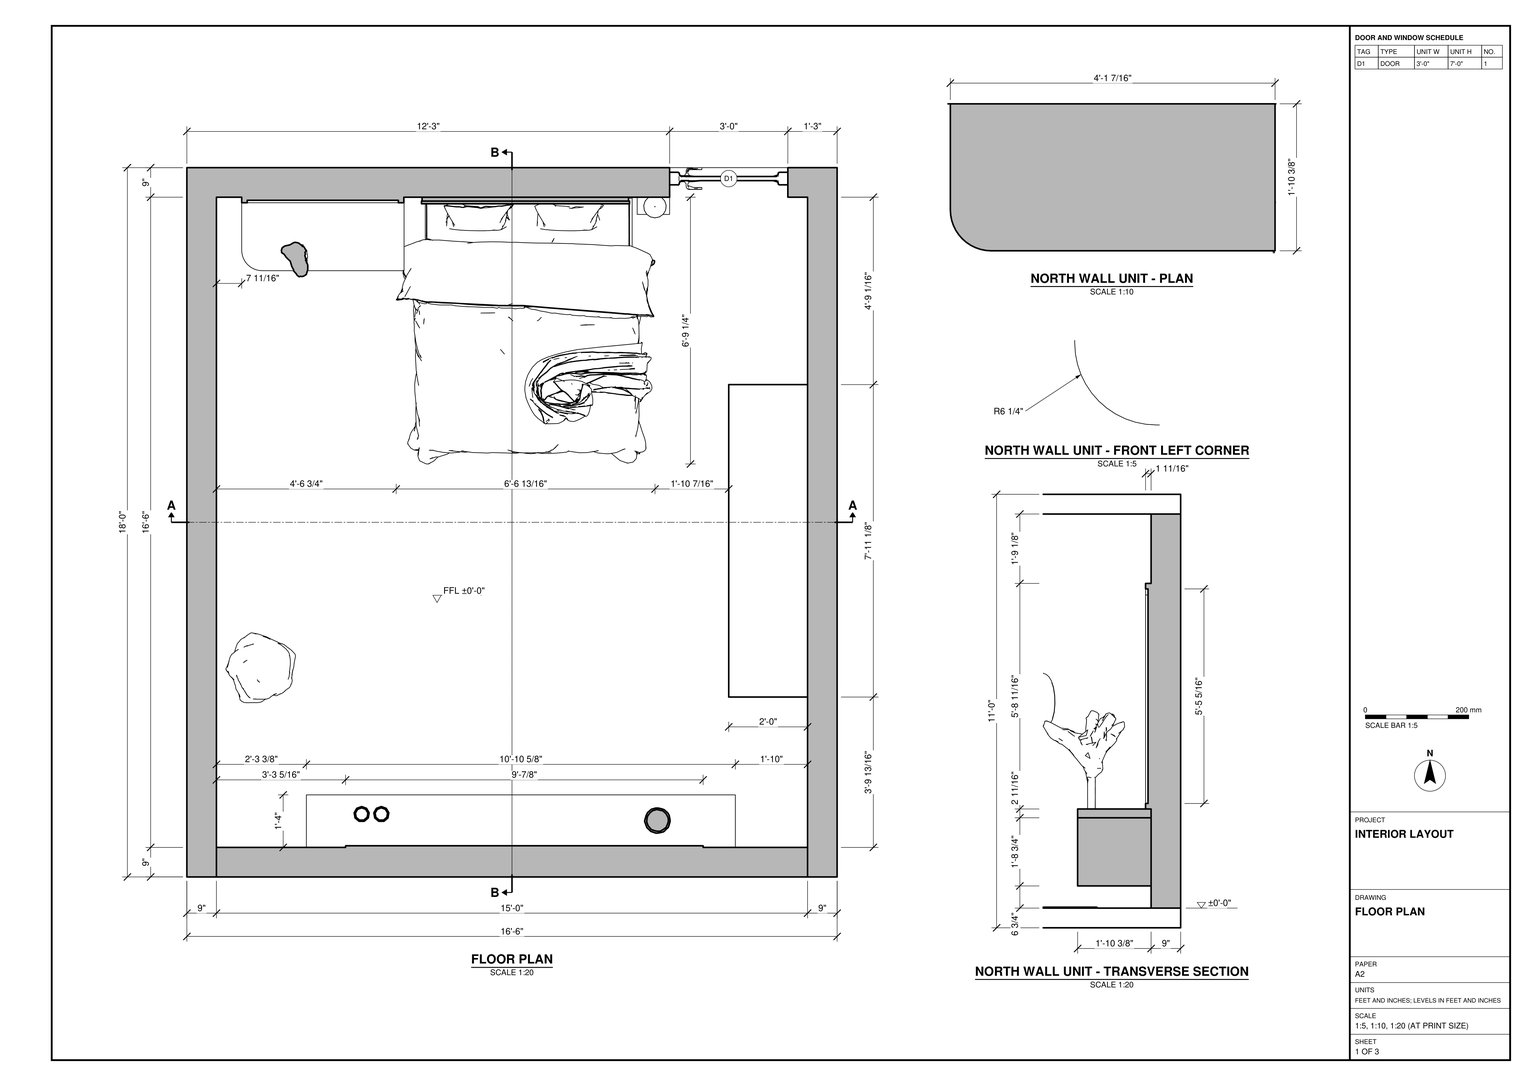
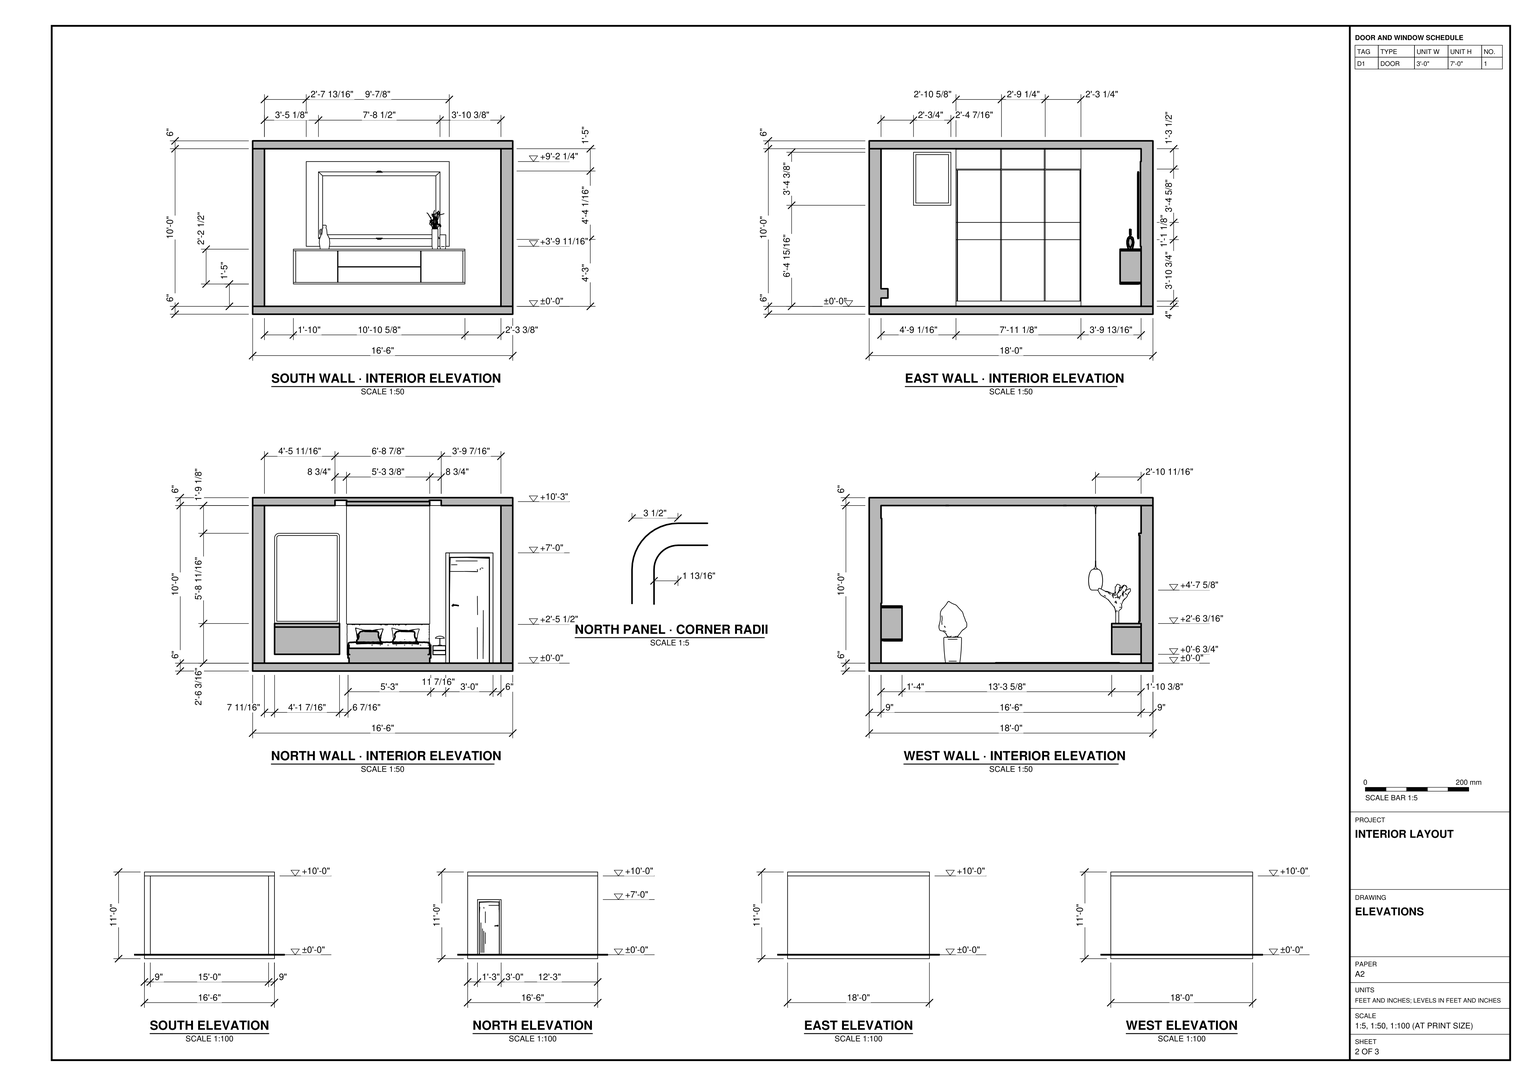
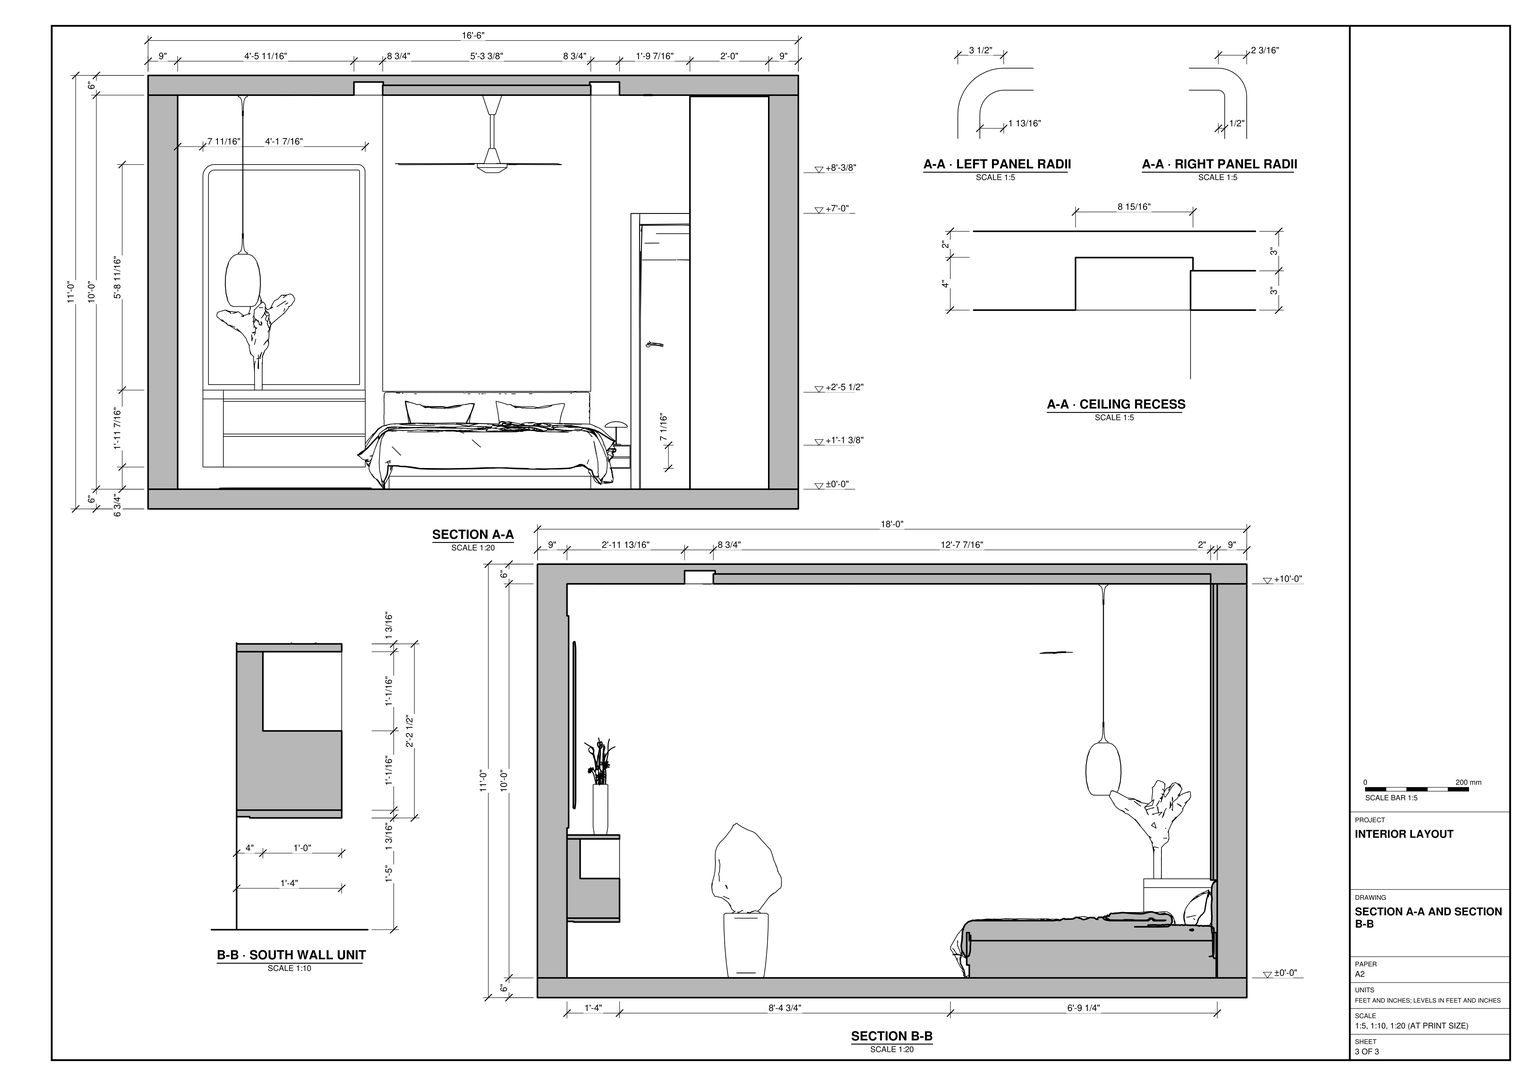
Build the bedroom in SketchUp from task_files/diagram_01.pdf. Work in feet and inches. The room shell measures 16'-6" east to west by 18'-0" north to south, with an overall height of 11'-0". Use the finished floor at ±0'-0" as the single storey level. Model the 9" perimeter walls, the 6" floor and roof slabs, and the stepped recess in the ceiling shown in sections A-A and B-B. Place the 3'-0" by 7'-0" entrance door near the east end of the north wall.

Set the platform bed with its head against the north wall. Align the tall panel behind the headboard with the ceiling detail. To the left of the bed, model the suspended cabinet with its rounded front-left corner and the framed panel above it. Include the small bedside unit on the door side. Use the east elevation to lay out the divisions on the full-height storage unit. Opposite the bed, model the floating south wall cabinet with its shelving and the framed rectangular panel above it. Place the ceiling fan, pendant, floor plant and tabletop objects where shown. Decor and loose items may be any suitable library components.

Keep the walls, floor slab and roof separate, and make each furniture or joinery piece a separate group or component. Use components for repeated parts. Save one SketchUp model as output_files/bedroom_with_fitted_wall_units_and_a_recessed_ceiling.skp.

# SketchUp Ruby script. Lengths in inches.
U = 1.inch
M = Sketchup.active_model
def pt(a) = Geom::Point3d.new(a.map { |v| v * U })
def face(e, loops, mat)
  f = e.add_face(loops[0].map { |a| pt(a) })
  loops[1..].each { |l| e.add_face(l.map { |a| pt(a) }).erase! }
  f.material = f.back_material = mat if mat
  f
end
# faces: each face lists its corners as indices into pts; further lists are holes
def faces(e, pts, list, mat = nil) = list.each { |f| face(e, (f[0].is_a?(Array) ? f : [f]).map { |l| l.map { |i| pts[i] } }, mat) }
# xy, xz, yz: faces in a plane at the given z, y or x. An outline is a flat list of corners, or four numbers for a rectangle; further outlines are holes
def ring(l) = l.size == 4 ? [[l[0], l[1]], [l[2], l[1]], [l[2], l[3]], [l[0], l[3]]] : l.each_slice(2).to_a
def flat(e, list, mat, &to3) = list.each { |f| face(e, (f[0].is_a?(Array) ? f : [f]).map { |l| ring(l).map { |u, v| to3.(u, v) } }, mat) }
def xy(e, z, list, mat = nil) = flat(e, list, mat) { |x, y| [x, y, z] }
def xz(e, y, list, mat = nil) = flat(e, list, mat) { |x, z| [x, y, z] }
def yz(e, x, list, mat = nil) = flat(e, list, mat) { |y, z| [x, y, z] }
def lines(e, pts, list) = list.each { |a, b| e.add_line(pt(pts[a]), pt(pts[b])) }
# prism: a flat outline (further loops are holes) pulled along v
def prism(e, loops, v, mat = nil)
  f = face(e, loops, mat); d = Geom::Vector3d.new(v.map { |x| x * U })
  f.pushpull(f.normal.samedirection?(d) ? d.length : -d.length)
end
def box(e, o, s, mat = nil) = prism(e, [[o, [o[0] + s[0], o[1], o[2]], [o[0] + s[0], o[1] + s[1], o[2]], [o[0], o[1] + s[1], o[2]]]], [0, 0, s[2]], mat)
def at(x, y, z, deg = 0) = Geom::Transformation.translation(pt([x, y, z])) * Geom::Transformation.rotation(ORIGIN, Z_AXIS, deg.degrees)
def axes(o, x, y, z) = Geom::Transformation.new([*x, 0, *y, 0, *z, 0, *pt(o).to_a, 1])
def part(name) = M.definitions.add(name)
# library, detail: a bought-in or finely detailed component or shape, given as its bounding box
def library(name, o, s) = part(name).tap { |d| box(d.entities, o, s) }
def detail(e, o, s) = box(e.add_group.entities, o, s)
def put(e, d, t, mat = nil) = e.add_instance(d, t).tap { |i| i.material = mat if mat }
def group(e, t, mat = nil) = e.add_group.tap { |g| g.transformation = t; g.material = mat if mat }.entities
root = M.entities
M.materials.add("Emissive").color = [188, 188, 142]
M.materials.add("Generic").color = [137, 153, 144]
M.materials.add("Generic\#1").color = [189, 193, 187]
M.materials.add("Glass Mirror 001").color = [0, 0, 0]
M.materials["Glass Mirror 001"].alpha = 0.1
M.materials.add("Marble White 100cm").color = [221, 221, 221]
M.materials.add("W144X948F75_NILAYA EQUINOX FD25735 ROLL F75").color = [223, 227, 229]
M.materials.add("[Color M01]").color = [59, 22, 6]
M.materials.add("[Color M02]").color = [198, 198, 198]
c1 = library("bed",[0,0,0],[81.24,78.82,29.53])
c2 = library("Component4",[-334.86,-221.33,0],[669.72,442.66,2])
c3 = part("Group\#10")
g1 = group(c3.entities,at(1.62,23.48,0.37))
prism(g1,[[[2.19,-1.21,0],[0.78,-1.47,0],[-0.07,3.1,0],[1.34,3.36,0]]],[0,0,0.04])
g2 = group(c3.entities,at(0,0,0))
xy(g2,0.33,[[3.33,0,0,23.09,1.89,23.4375],[3.33,0,1.89,23.4375,2.83,23.62],[3.33,0,2.83,23.62,4.25,23.88,8.53,0.97,7.12,0.71]])
xy(g2,0.37,[[3.33,0,1.89,23.4375,0,23.09],[3.33,0,2.83,23.62,1.89,23.4375],[3.33,0,7.12,0.71,8.53,0.97,4.25,23.88,2.83,23.62]])
p = [[5.64,24.14,0.12],[4.25,23.88,0.37],[8.53,0.97,0.37],[10.39,1.32,0.04],[4.25,23.88,0.33],[5.64,24.14,0.08],
  [10.39,1.32,0],[8.53,0.97,0.33],[2.83,23.62,0.33],[1.89,23.4375,0.33],[0,23.09,0.33],[0,23.09,0.37],
  [1.89,23.4375,0.37],[2.83,23.62,0.37],[3.33,0,0.33],[3.33,0,0.37],[7.12,0.71,0.37],[7.12,0.71,0.33]]
faces(g2,p,[[0,1,2,3],[4,5,6,7],[6,3,2,7],[5,0,3,6],[0,5,4,8,9,10,11,12,13,1],[14,15,11,10],[7,2,16,15,14,17]])
c4 = part("ceiling fan")
g3 = group(c4.entities,at(0.63,30.3,-2.8,-91.2))
g4 = group(g3,at(24.19,24.96,0))
xy(g4,0,[[4.53,2.58,4.03,2.65,3.56,2.84,3.16,3.15,2.85,3.55,2.65,4.02,2.58,4.52,2.65,5.02,2.84,5.5,3.15,5.9,3.55,6.21,4.02,6.41,4.52,6.47,5.02,6.41,5.5,6.22,5.9,5.91,6.21,5.51,6.41,5.04,6.47,4.53,6.41,4.03,6.22,3.56,5.91,3.16,5.51,2.85,5.04,2.65]])
xy(g4,2.76,[[4.54,0,5.71,0.16,6.8,0.61,7.74,1.34,8.46,2.28,8.9,3.37,9.06,4.54,8.9,5.71,8.44,6.8,7.72,7.74,6.78,8.46,5.68,8.9,4.51,9.06,3.34,8.9,2.25,8.44,1.32,7.72,0.6,6.78,0.15,5.68,0,4.51,0.16,3.34,0.61,2.25,1.34,1.32,2.28,0.6,3.37,0.15]])
p = [[4.54,0,1.57],[3.37,0.15,1.57],[4.03,2.65,0],[4.53,2.58,0],[5.71,0.16,1.57],[5.04,2.65,0],
  [2.28,0.6,1.57],[3.56,2.84,0],[6.8,0.61,1.57],[5.51,2.85,0],[1.34,1.32,1.57],[3.16,3.15,0],
  [7.74,1.34,1.57],[5.91,3.16,0],[0.61,2.25,1.57],[2.85,3.55,0],[8.46,2.28,1.57],[6.22,3.56,0],
  [0.16,3.34,1.57],[2.65,4.02,0],[8.9,3.37,1.57],[6.41,4.03,0],[0,4.51,1.57],[2.58,4.52,0],
  [9.06,4.54,1.57],[6.47,4.53,0],[0.15,5.68,1.57],[2.65,5.02,0],[8.9,5.71,1.57],[6.41,5.04,0],
  [0.6,6.78,1.57],[2.84,5.5,0],[8.44,6.8,1.57],[6.21,5.51,0],[1.32,7.72,1.57],[3.15,5.9,0],
  [7.72,7.74,1.57],[5.9,5.91,0],[2.25,8.44,1.57],[3.55,6.21,0],[6.78,8.46,1.57],[5.5,6.22,0],
  [3.34,8.9,1.57],[4.02,6.41,0],[5.68,8.9,1.57],[5.02,6.41,0],[4.51,9.06,1.57],[4.52,6.47,0],
  [3.37,0.15,2.76],[4.54,0,2.76],[5.71,0.16,2.76],[2.28,0.6,2.76],[6.8,0.61,2.76],[1.34,1.32,2.76],
  [7.74,1.34,2.76],[0.61,2.25,2.76],[8.46,2.28,2.76],[0.16,3.34,2.76],[8.9,3.37,2.76],[0,4.51,2.76],
  [9.06,4.54,2.76],[0.15,5.68,2.76],[8.9,5.71,2.76],[0.6,6.78,2.76],[8.44,6.8,2.76],[1.32,7.72,2.76],
  [7.72,7.74,2.76],[2.25,8.44,2.76],[6.78,8.46,2.76],[3.34,8.9,2.76],[5.68,8.9,2.76],[4.51,9.06,2.76]]
faces(g4,p,[[0,1,2,3],[4,0,3,5],[1,6,7,2],[8,4,5,9],[6,10,11,7],[12,8,9,13],[10,14,15,11],[16,12,13,17],
  [14,18,19,15],[20,16,17,21],[18,22,23,19],[24,20,21,25],[22,26,27,23],[28,24,25,29],[26,30,31,27],[32,28,29,33],
  [30,34,35,31],[36,32,33,37],[34,38,39,35],[40,36,37,41],[38,42,43,39],[44,40,41,45],[42,46,47,43],[46,44,45,47],
  [48,1,0,49],[49,0,4,50],[51,6,1,48],[50,4,8,52],[53,10,6,51],[52,8,12,54],[55,14,10,53],[54,12,16,56],
  [57,18,14,55],[56,16,20,58],[59,22,18,57],[58,20,24,60],[61,26,22,59],[60,24,28,62],[63,30,26,61],[62,28,32,64],
  [65,34,30,63],[64,32,36,66],[67,38,34,65],[66,36,40,68],[69,42,38,67],[68,40,44,70],[71,46,42,69],[70,44,46,71]])
put(g3,c3,at(26.98,0,2.42))
put(g3,c3,at(4.05,45.73,2.42,-120))
put(g3,c3,at(55.12,42.72,2.42,120))
g5 = group(g3,at(25.76,26.53,17.72))
p = [[2.95,2.95,7.28],[2.95,2.95,5.91]]
lines(g5,p,[[0,1]])
g6 = group(g5,at(0,0,5.91))
xy(g6,-5.91,[[[2.95,1.99,2.7,2.02,2.47,2.12,2.27,2.27,2.12,2.47,2.02,2.7,1.99,2.95,2.02,3.2,2.12,3.4375,2.27,3.64,2.47,3.79,2.7,3.89,2.95,3.92,3.2,3.89,3.4375,3.79,3.64,3.64,3.79,3.4375,3.89,3.2,3.92,2.95,3.89,2.7,3.79,2.47,3.64,2.27,3.4375,2.12,3.2,2.02],[2.95,2.38,3.1,2.4,3.24,2.46,3.36,2.55,3.45,2.67,3.5,2.81,3.52,2.95,3.5,3.1,3.45,3.24,3.36,3.36,3.24,3.45,3.1,3.5,2.95,3.52,2.81,3.5,2.67,3.45,2.55,3.36,2.46,3.24,2.4,3.1,2.38,2.95,2.4,2.81,2.46,2.67,2.55,2.55,2.67,2.46,2.81,2.4]]])
xy(g6,0,[[2.95,0,3.72,0.1,4.43,0.4,5.04,0.86,5.51,1.48,5.8,2.1875,5.91,2.95,5.8,3.72,5.51,4.43,5.04,5.04,4.43,5.51,3.72,5.8,2.95,5.91,2.1875,5.8,1.48,5.51,0.86,5.04,0.4,4.43,0.1,3.72,0,2.95,0.1,2.1875,0.4,1.48,0.86,0.86,1.48,0.4,2.1875,0.1]])
p = [[2.95,0,0],[2.1875,0.1,0],[2.7,2.02,-5.91],[2.95,1.99,-5.91],[3.72,0.1,0],[3.2,2.02,-5.91],
  [1.48,0.4,0],[2.47,2.12,-5.91],[4.43,0.4,0],[3.4375,2.12,-5.91],[0.86,0.86,0],[2.27,2.27,-5.91],
  [5.04,0.86,0],[3.64,2.27,-5.91],[0.4,1.48,0],[2.12,2.47,-5.91],[5.51,1.48,0],[3.79,2.47,-5.91],
  [0.1,2.1875,0],[2.02,2.7,-5.91],[5.8,2.1875,0],[3.89,2.7,-5.91],[0,2.95,0],[1.99,2.95,-5.91],
  [5.91,2.95,0],[3.92,2.95,-5.91],[0.1,3.72,0],[2.02,3.2,-5.91],[5.8,3.72,0],[3.89,3.2,-5.91],
  [0.4,4.43,0],[2.12,3.4375,-5.91],[5.51,4.43,0],[3.79,3.4375,-5.91],[0.86,5.04,0],[2.27,3.64,-5.91],
  [5.04,5.04,0],[3.64,3.64,-5.91],[1.48,5.51,0],[2.47,3.79,-5.91],[4.43,5.51,0],[3.4375,3.79,-5.91],
  [2.1875,5.8,0],[2.7,3.89,-5.91],[3.72,5.8,0],[3.2,3.89,-5.91],[2.95,5.91,0],[2.95,3.92,-5.91]]
faces(g6,p,[[0,1,2,3],[4,0,3,5],[1,6,7,2],[8,4,5,9],[6,10,11,7],[12,8,9,13],[10,14,15,11],[16,12,13,17],
  [14,18,19,15],[20,16,17,21],[18,22,23,19],[24,20,21,25],[22,26,27,23],[28,24,25,29],[26,30,31,27],[32,28,29,33],
  [30,34,35,31],[36,32,33,37],[34,38,39,35],[40,36,37,41],[38,42,43,39],[44,40,41,45],[42,46,47,43],[46,44,45,47]])
g7 = group(g3,at(25.76,26.53,1.46))
xy(g7,0,[[2.95,0,3.72,0.1,4.43,0.4,5.04,0.86,5.51,1.48,5.8,2.1875,5.91,2.95,5.8,3.72,5.51,4.43,5.04,5.04,4.43,5.51,3.72,5.8,2.95,5.91,2.1875,5.8,1.48,5.51,0.86,5.04,0.4,4.43,0.1,3.72,0,2.95,0.1,2.1875,0.4,1.48,0.86,0.86,1.48,0.4,2.1875,0.1]])
xy(g7,5.91,[[[2.95,1.99,2.7,2.02,2.47,2.12,2.27,2.27,2.12,2.47,2.02,2.7,1.99,2.95,2.02,3.2,2.12,3.4375,2.27,3.64,2.47,3.79,2.7,3.89,2.95,3.92,3.2,3.89,3.4375,3.79,3.64,3.64,3.79,3.4375,3.89,3.2,3.92,2.95,3.89,2.7,3.79,2.47,3.64,2.27,3.4375,2.12,3.2,2.02],[2.95,2.38,3.1,2.4,3.24,2.46,3.36,2.55,3.45,2.67,3.5,2.81,3.52,2.95,3.5,3.1,3.45,3.24,3.36,3.36,3.24,3.45,3.1,3.5,2.95,3.52,2.81,3.5,2.67,3.45,2.55,3.36,2.46,3.24,2.4,3.1,2.38,2.95,2.4,2.81,2.46,2.67,2.55,2.55,2.67,2.46,2.81,2.4]]])
p = [[2.95,0,0],[2.1875,0.1,0],[2.7,2.02,5.91],[2.95,1.99,5.91],[3.72,0.1,0],[3.2,2.02,5.91],
  [1.48,0.4,0],[2.47,2.12,5.91],[4.43,0.4,0],[3.4375,2.12,5.91],[0.86,0.86,0],[2.27,2.27,5.91],
  [5.04,0.86,0],[3.64,2.27,5.91],[0.4,1.48,0],[2.12,2.47,5.91],[5.51,1.48,0],[3.79,2.47,5.91],
  [0.1,2.1875,0],[2.02,2.7,5.91],[5.8,2.1875,0],[3.89,2.7,5.91],[0,2.95,0],[1.99,2.95,5.91],
  [5.91,2.95,0],[3.92,2.95,5.91],[0.1,3.72,0],[2.02,3.2,5.91],[5.8,3.72,0],[3.89,3.2,5.91],
  [0.4,4.43,0],[2.12,3.4375,5.91],[5.51,4.43,0],[3.79,3.4375,5.91],[0.86,5.04,0],[2.27,3.64,5.91],
  [5.04,5.04,0],[3.64,3.64,5.91],[1.48,5.51,0],[2.47,3.79,5.91],[4.43,5.51,0],[3.4375,3.79,5.91],
  [2.1875,5.8,0],[2.7,3.89,5.91],[3.72,5.8,0],[3.2,3.89,5.91],[2.95,5.91,0],[2.95,3.92,5.91]]
faces(g7,p,[[0,1,2,3],[4,0,3,5],[1,6,7,2],[8,4,5,9],[6,10,11,7],[12,8,9,13],[10,14,15,11],[16,12,13,17],
  [14,18,19,15],[20,16,17,21],[18,22,23,19],[24,20,21,25],[22,26,27,23],[28,24,25,29],[26,30,31,27],[32,28,29,33],
  [30,34,35,31],[36,32,33,37],[34,38,39,35],[40,36,37,41],[38,42,43,39],[44,40,41,45],[42,46,47,43],[46,44,45,47]])
g8 = group(g3,at(25.76,26.53,27.76))
prism(g8,[[[2.95,2.38,-20.39],[2.81,2.4,-20.39],[2.67,2.46,-20.39],[2.55,2.55,-20.39],[2.46,2.67,-20.39],[2.4,2.81,-20.39],[2.38,2.95,-20.39],[2.4,3.1,-20.39],[2.46,3.24,-20.39],[2.55,3.36,-20.39],[2.67,3.45,-20.39],[2.81,3.5,-20.39],[2.95,3.52,-20.39],[3.1,3.5,-20.39],[3.24,3.45,-20.39],[3.36,3.36,-20.39],[3.45,3.24,-20.39],[3.5,3.1,-20.39],[3.52,2.95,-20.39],[3.5,2.81,-20.39],[3.45,2.67,-20.39],[3.36,2.55,-20.39],[3.24,2.46,-20.39],[3.1,2.4,-20.39]]],[0,0,10.35])
c5 = library("Tlon Light 1350 Ceiling 152 009",[-26.57,-26.57,-3.78],[53.14,53.14,3.72])
c6 = library("Potted Plant 60-25",[-10.7,-10.47,0],[21.2,21.27,47.12])
c7 = library("Pendant 16-40",[-13.91,-13.91,-52.32],[27.82,27.82,52.32])
c8 = library("Takayama Table Lamp",[-8.62,-8.67,-0.01],[17.24,19.8,18.21])
c9 = library("Door 243 039",[-21.61,-3.32,0],[43.22,6.64,82.63])
c10 = library("Vase 293 015",[-12.68,-14.72,0],[23.75,24.8,29.92])
c11 = library("Vase 296 003 004",[-4.05,-3.96,-0.125],[8.06,7.98,18.4])
c12 = library("Vases 103-09",[-7.17,-4.68,0],[14.43,9.35,29.62])
c13 = library("Flat screen television",[0,1.41,1.14],[35.92,0.28,20.21])
xy(root,-6,[[0,0,198,216]])
xy(root,0,[[0,0,9,0,9,207,147,207,147,216,0,216],[9,0,189,9],[189,0,198,0,198,216,183,216,183,207,189,207],[165,54.79,189,149.93]])
xy(root,0,[[9,9,189,9,189,54.79,165,54.79,165,149.93,189,149.93,189,207,183,207,183,216,147,216,147,207,9,207]],"Marble White 100cm")
xy(root,6.34,[[137.125,201.75,147,207]])
xy(root,6.75,[[22.93,184.625,22.11,184.68,21.3125,184.84,20.54,185.1,19.8125,185.46,19.13,185.91,18.52,186.45,17.99,187.0625,17.53,187.74,17.17,188.47,16.91,189.24,16.75,190.04,16.7,190.85,16.7,207,66.14,207,66.14,184.625]],"Generic\#1")
xy(root,13.4,[[137.125,201.75,147,207]],"Generic\#1")
xy(root,17.02,[[36.39,11,167.01,25]])
xy(root,17.2,[[36.39,9,167.01,11]],"Emissive")
xy(root,18.2,[[36.39,9,167.01,25]])
xy(root,27.5,[[22.93,184.625,22.11,184.68,21.3125,184.84,20.54,185.1,19.8125,185.46,19.13,185.91,18.52,186.45,17.99,187.0625,17.53,187.74,17.17,188.47,16.91,189.24,16.75,190.04,16.7,190.85,16.7,207,66.14,207,66.14,184.625]])
xy(root,29.81,[[71.4375,205,134.8,205.8125],[71.625,205.8125,134.49,207]])
xy(root,30.18,[[16.7,205.3125,66.07,207]])
xy(root,30.18,[[22.93,184.625,66.14,184.625,66.14,207,66.07,207,66.07,205.3125,16.7,205.3125,16.7,190.85,16.75,190.04,16.91,189.24,17.17,188.47,17.53,187.74,17.99,187.0625,18.52,186.45,19.13,185.91,19.8125,185.46,20.54,185.1,21.3125,184.84,22.11,184.68]],"Generic\#1")
xy(root,30.27,[[70.16,13,132.99,25]],"Generic")
xy(root,31.86,[[18.375,205.3125,64.4,206.0625]],"Generic")
xy(root,42.33,[[36.39,9,36.39,25,70.16,25,70.16,13,132.99,13,132.99,25,167.01,25,167.01,9]])
xy(root,42.33,[[70.16,13,132.99,25]],"Generic")
xy(root,43.52,[[36.39,9,167.01,25]])
xy(root,45.68,[[48.33,9,157.2,9.5]],"Emissive")
xy(root,76.92,[[188.625,153.82,189,182.26]])
xy(root,78.68,[[188.625,155.59,188.875,180.5]])
xy(root,84,[[147,207,183,216]],"Generic")
xy(root,97.2,[[20.21,205.3125,63.9,206.0625]],"Generic")
xy(root,98.87,[[20.21,205.3125,63.9,207]],"Generic")
xy(root,110.24,[[48.33,9,157.2,9.5]],"Emissive")
xy(root,115.53,[[188.625,155.59,188.875,180.5]])
xy(root,117.3,[[188.625,153.82,189,182.26]])
xy(root,119.6,[[165,54.79,189,149.93]])
xy(root,120,[[0,0,0,216,198,216,198,0,189,0,189,207,143.55,207,143.55,213.75,62.68,213.75,62.68,207,9,207,9,0],[9,9,9,207,62.68,207,62.68,44.81,143.55,44.81,143.55,207,189,207,189,149.93,165,149.93,165,54.79,189,54.79,189,9],[165,54.79,189,149.93],[71.4375,205,134.8,205.8125],[71.625,205.8125,134.49,207],
  [62.68,207,143.55,213.75]])
xy(root,120,[[71.4375,53.5625,134.8,205]],"W144X948F75_NILAYA EQUINOX FD25735 ROLL F75")
xy(root,123,[[71.625,54.125,134.49,205]])
xy(root,123,[[71.4375,53.5625,71.625,205],[71.625,53.5625,134.49,54.125],[134.49,53.5625,134.8,205],[71.4375,205,71.625,205.95],[134.49,205,134.8,205.8125]],"Emissive")
xy(root,124,[[62.68,44.81,62.68,207,71.625,207,71.625,54.125,134.49,54.125,134.49,207,143.55,207,143.55,44.81]])
xy(root,126,[[0,0,198,216]])
xz(root,0,[[0,-6,198,0],[0,0,9,120],[9,0,189,120],[189,0,198,120],[0,120,198,126]])
xz(root,9,[[[9,0,189,120],[48.33,45.68,157.2,110.24],[36.39,17.2,167.01,43.52]],[36.39,17.2,167.01,18.2],[36.39,18.2,167.01,42.33],[36.39,42.33,167.01,43.52]])
xz(root,9.5,[[48.33,45.68,157.2,110.24]])
xz(root,11,[[36.39,17.02,167.01,17.2]],"Emissive")
xz(root,13,[[70.16,30.27,132.99,42.33]],"Generic")
xz(root,25,[[36.39,17.02,167.01,18.2],[36.39,18.2,37.95,42.33],[165.2,18.2,167.01,42.33],[36.39,42.33,167.01,43.52]])
xz(root,25,[[37.95,18.2,69.76,42.33],[69.76,18.2,70.16,42.33],[70.16,18.2,132.99,30.27],[132.99,18.2,133.39,42.33],[133.39,18.2,165.2,42.33]],"Generic")
xz(root,44.81,[[62.68,120,143.55,124]])
xz(root,53.5625,[[71.4375,120,134.8,123]])
xz(root,54.125,[[71.625,123,134.49,124]],"Emissive")
xz(root,54.79,[[165,119.6,189,120]])
xz(root,54.79,[[165,0,189,119.6]],"Generic\#1")
xz(root,149.93,[[165,119.6,189,120]])
xz(root,149.93,[[165,0,189,119.6]],"Generic\#1")
xz(root,153.82,[[188.625,76.92,189,117.3]])
xz(root,155.59,[[188.625,78.68,188.875,115.53]])
xz(root,180.5,[[188.625,78.68,188.875,115.53]])
xz(root,182.26,[[188.625,76.92,189,117.3]])
xz(root,184.625,[[22.93,6.75,66.14,16.06],[22.93,16.06,66.14,16.81],[22.93,16.81,66.14,26.75],[22.93,26.75,66.14,27.5]],"Generic")
xz(root,184.625,[[22.93,27.5,66.14,30.18]],"Generic\#1")
xz(root,201.75,[[[137.125,6.34,147,13.4],[137.39,6.6,146.74,13.14]],[137.39,6.6,146.74,9.47],[137.39,9.47,146.74,9.87],[137.39,9.87,146.74,13.14]],"Generic")
xz(root,205,[[71.4375,120,134.8,123]])
xz(root,205,[[71.4375,29.81,134.8,120]],"W144X948F75_NILAYA EQUINOX FD25735 ROLL F75")
xz(root,205.3125,[[[16.7,30.18,66.07,30.18,66.07,96.7,66.06,96.98,66,97.26,65.91,97.53,65.78,97.78,65.625,98.02,65.4375,98.23,65.22,98.42,64.99,98.58,64.73,98.71,64.46,98.8,64.18,98.85,63.9,98.87,20.21,98.87,19.75,98.84,19.3,98.75,18.87,98.6,18.45,98.4,18.07,98.15,17.73,97.84,17.42,97.5,17.17,97.12,16.97,96.7,16.82,96.27,16.73,95.82,16.7,95.36],[18.375,31.86,18.375,95.36,18.39,95.6,18.4375,95.84,18.51,96.0625,18.62,96.28,18.75,96.48,18.91,96.66,19.09,96.82,19.29,96.95,19.51,97.06,19.73,97.13,19.97,97.18,20.21,97.2,63.9,97.2,63.96,97.19,64.03,97.18,64.09,97.16,64.15,97.13,64.25,97.05,64.33,96.95,64.36,96.89,64.38,96.83,64.39,96.76,64.4,96.7,64.4,31.86]]],"Generic")
xz(root,205.8125,[[71.625,29.81,134.49,120]])
xz(root,205.8125,[[71.4375,29.81,71.625,120],[134.49,29.81,134.8,120],[134.49,120,134.8,123]],"Emissive")
xz(root,206.0625,[[18.375,31.86,64.4,31.86,64.4,96.7,64.39,96.76,64.38,96.83,64.36,96.89,64.33,96.95,64.25,97.05,64.15,97.13,64.09,97.16,64.03,97.18,63.96,97.19,63.9,97.2,20.21,97.2,19.97,97.18,19.73,97.13,19.51,97.06,19.29,96.95,19.09,96.82,18.91,96.66,18.75,96.48,18.62,96.28,18.51,96.0625,18.4375,95.84,18.39,95.6,18.375,95.36]],"Glass Mirror 001")
xz(root,207,[[[9,0,147,0,147,6.34,137.125,6.34,137.125,13.4,147,13.4,147,84,183,84,183,0,189,0,189,120,134.49,120,134.49,29.81,71.625,29.81,71.625,120,9,120],[16.7,6.75,16.7,95.36,16.73,95.82,16.82,96.27,16.97,96.7,17.17,97.12,17.42,97.5,17.73,97.84,18.07,98.15,18.45,98.4,18.87,98.6,19.3,98.75,19.75,98.84,20.21,98.87,63.9,98.87,64.18,98.85,64.46,98.8,64.73,98.71,64.99,98.58,65.22,98.42,65.4375,98.23,65.625,98.02,65.78,97.78,65.91,97.53,66,97.26,66.06,96.98,66.07,96.7,66.07,30.18,66.14,30.18,66.14,6.75]],[16.7,6.75,66.14,27.5],[16.7,27.5,66.14,30.18],[71.625,29.81,134.49,120],[62.68,120,71.625,124],
  [134.49,120,143.55,124]])
xz(root,216,[[0,-6,198,0],[0,0,0,120,198,120,198,0,183,0,183,84,147,84,147,0],[0,120,198,126]])
yz(root,0,[[0,-6,216,0],[0,0,216,120],[0,120,216,126]])
yz(root,9,[[0,0,9,120],[9,0,207,120]])
yz(root,16.7,[[205.3125,30.18,207,95.36]])
yz(root,16.7,[[190.85,6.75,207,27.5],[190.85,27.5,207,30.18]],"Generic\#1")
yz(root,18.375,[[205.3125,31.86,206.0625,95.36]],"Generic")
yz(root,36.39,[[11,17.02,11,17.2,9,17.2,9,18.2,25,18.2,25,17.02],[9,18.2,25,42.33],[9,42.33,25,43.52]])
yz(root,48.33,[[9,45.68,9.5,110.24]],"Emissive")
yz(root,62.68,[[44.81,120,207,124]])
yz(root,64.4,[[205.3125,31.86,206.0625,96.7]],"Generic")
yz(root,66.07,[[205.3125,30.18,207,96.7]],"Generic")
yz(root,66.14,[[184.625,6.75,207,27.5],[184.625,27.5,207,30.18]],"Generic")
yz(root,70.16,[[13,30.27,25,42.33]],"Generic")
yz(root,71.4375,[[205,29.81,205.8125,120],[53.5625,120,205,123],[205,120,205,123,205.95,123,205.8125,120]])
yz(root,71.625,[[205.8125,29.81,207,120],[205.8125,120,205.95,123,206,124,207,124,207,120],[54.125,123,205,124],[205,123,205,124,206,124,205.95,123]],"Emissive")
yz(root,132.99,[[13,30.27,25,42.33]],"Generic")
yz(root,134.49,[[205.8125,29.81,207,120],[205.8125,120,207,124],[54.125,123,205,124],[205,123,205.8125,124]],"Emissive")
yz(root,134.8,[[205,29.81,205.8125,120],[53.5625,120,205,123],[205,120,205.8125,123]])
yz(root,137.125,[[201.75,6.34,207,13.4]])
yz(root,143.55,[[44.81,120,207,124]])
yz(root,147,[[207,0,216,0,216,84,207,84,207,13.4,201.75,13.4,201.75,6.34,207,6.34]],"Generic")
yz(root,157.2,[[9,45.68,9.5,110.24]],"Emissive")
yz(root,165,[[115.28,4,116.03,50.77]])
yz(root,165,[[55.59,50.77,82.01,63.87],[82.01,50.77,82.76,63.87],[82.76,50.77,115.28,63.87],[115.28,50.77,116.03,63.87],[116.03,50.77,148.72,63.87],
  [148.72,50.77,149.12,63.87],[149.12,50.77,149.93,63.87]],"Generic")
yz(root,165,[[54.79,0,149.93,4],[54.79,4,55.1875,103.74],[55.1875,4,55.59,50.77],[55.59,4,82.01,50.77],[82.01,4,82.76,50.77],
  [82.76,4,115.28,50.77],[116.03,4,148.72,50.77],[148.72,4,149.12,50.77],[149.12,4,149.93,50.77],[55.1875,50.77,55.59,63.87],
  [55.1875,63.87,55.59,103.74],[55.59,63.87,82.01,103.74],[82.01,63.87,82.76,103.74],[82.76,63.87,115.28,103.74],[115.28,63.87,116.03,103.74],
  [116.03,63.87,148.72,103.74],[148.72,63.87,149.12,103.74],[149.12,63.87,149.93,103.74],[54.79,103.74,82.76,104.49],[82.76,103.74,116.03,104.49],
  [116.03,103.74,149.93,104.49],[54.79,104.49,82.01,119.6],[82.01,104.49,82.76,119.6],[82.76,104.49,115.28,119.6],[115.28,104.49,116.03,119.6],
  [116.03,104.49,149.93,119.6],[54.79,119.6,149.93,120]],"Generic\#1")
yz(root,167.01,[[11,17.02,25,17.02,25,18.2,9,18.2,9,17.2,11,17.2],[9,18.2,25,42.33],[9,42.33,25,43.52]])
yz(root,183,[[207,0,216,84]],"Generic")
yz(root,188.625,[[[153.82,76.92,182.26,117.3],[155.59,78.68,180.5,115.53]]],"[Color M02]")
yz(root,188.875,[[155.59,78.68,180.5,115.53]],"[Color M01]")
yz(root,189,[[0,0,9,120],[9,0,54.79,120],[54.79,0,149.93,119.6],[[149.93,0,207,120],[153.82,76.92,182.26,117.3]],[54.79,119.6,149.93,120]])
yz(root,198,[[0,-6,216,0],[0,0,216,120],[0,120,216,126]])
p = [[22.93,184.625,26.75],[22.93,184.625,27.5],[22.11,184.68,27.5],[22.11,184.68,6.75],[22.93,184.625,6.75],[22.93,184.625,16.06],
  [22.93,184.625,16.81],[21.3125,184.84,27.5],[21.3125,184.84,6.75],[20.54,185.1,27.5],[20.54,185.1,6.75],[19.8125,185.46,27.5],
  [19.8125,185.46,6.75],[19.13,185.91,27.5],[19.13,185.91,6.75],[18.52,186.45,27.5],[18.52,186.45,6.75],[17.99,187.0625,27.5],
  [17.99,187.0625,6.75],[17.53,187.74,27.5],[17.53,187.74,6.75],[17.17,188.47,27.5],[17.17,188.47,6.75],[16.91,189.24,27.5],
  [16.91,189.24,6.75],[16.75,190.04,27.5],[16.75,190.04,6.75],[16.7,190.85,27.5],[16.7,190.85,6.75],[22.93,184.625,30.18],
  [22.11,184.68,30.18],[21.3125,184.84,30.18],[20.54,185.1,30.18],[19.8125,185.46,30.18],[19.13,185.91,30.18],[18.52,186.45,30.18],
  [17.99,187.0625,30.18],[17.53,187.74,30.18],[17.17,188.47,30.18],[16.91,189.24,30.18],[16.75,190.04,30.18],[16.7,190.85,30.18],
  [16.73,207,95.82],[16.7,207,95.36],[16.7,205.3125,95.36],[16.73,205.3125,95.82],[18.39,205.3125,95.6],[18.375,205.3125,95.36],
  [18.375,206.0625,95.36],[18.39,206.0625,95.6],[18.4375,205.3125,95.84],[18.4375,206.0625,95.84],[16.82,207,96.27],[16.82,205.3125,96.27],
  [18.51,205.3125,96.0625],[18.51,206.0625,96.0625],[18.62,205.3125,96.28],[18.62,206.0625,96.28],[16.97,207,96.7],[16.97,205.3125,96.7],
  [18.75,205.3125,96.48],[18.75,206.0625,96.48],[18.91,205.3125,96.66],[18.91,206.0625,96.66],[17.17,207,97.12],[17.17,205.3125,97.12],
  [19.09,205.3125,96.82],[19.09,206.0625,96.82],[64.4,205.3125,96.7],[64.39,205.3125,96.76],[64.39,206.0625,96.76],[64.4,206.0625,96.7],
  [66.07,207,96.7],[66.06,207,96.98],[66.06,205.3125,96.98],[66.07,205.3125,96.7],[19.29,205.3125,96.95],[19.29,206.0625,96.95],
  [64.38,205.3125,96.83],[64.38,206.0625,96.83],[64.36,205.3125,96.89],[64.36,206.0625,96.89],[19.51,205.3125,97.06],[19.51,206.0625,97.06],
  [64.33,205.3125,96.95],[64.33,206.0625,96.95],[64.29,205.3125,97],[64.29,206.0625,97],[64.25,205.3125,97.05],[64.2,205.3125,97.09],
  [64.2,206.0625,97.09],[64.25,206.0625,97.05],[66,207,97.26],[66,205.3125,97.26],[17.42,207,97.5],[17.42,205.3125,97.5],
  [19.73,205.3125,97.13],[19.73,206.0625,97.13],[19.97,205.3125,97.18],[19.97,206.0625,97.18],[64.15,205.3125,97.13],[64.15,206.0625,97.13],
  [64.09,205.3125,97.16],[64.09,206.0625,97.16],[20.21,205.3125,97.2],[20.21,206.0625,97.2],[63.96,205.3125,97.19],[63.9,205.3125,97.2],
  [63.9,206.0625,97.2],[63.96,206.0625,97.19],[64.03,205.3125,97.18],[64.03,206.0625,97.18],[65.91,207,97.53],[65.91,205.3125,97.53],
  [17.73,207,97.84],[17.73,205.3125,97.84],[65.78,207,97.78],[65.78,205.3125,97.78],[18.07,207,98.15],[18.07,205.3125,98.15],
  [65.625,207,98.02],[65.625,205.3125,98.02],[65.4375,207,98.23],[65.4375,205.3125,98.23],[18.45,207,98.4],[18.45,205.3125,98.4],
  [65.22,207,98.42],[65.22,205.3125,98.42],[18.87,207,98.6],[18.87,205.3125,98.6],[64.99,207,98.58],[64.99,205.3125,98.58],
  [19.3,207,98.75],[19.3,205.3125,98.75],[64.73,207,98.71],[64.73,205.3125,98.71],[64.46,207,98.8],[64.46,205.3125,98.8],
  [19.75,207,98.84],[19.75,205.3125,98.84],[20.21,207,98.87],[20.21,205.3125,98.87],[64.18,207,98.85],[64.18,205.3125,98.85],
  [63.9,207,98.87],[63.9,205.3125,98.87],[71.4375,205.8125,120],[71.4375,205.95,123],[71.625,205.95,123],[71.625,205.8125,120],
  [133.05,25,29.87],[132.99,25,29.87],[70.23,25,29.87]]
faces(root,p,[[0,1,2,3,4,5,6],[3,2,7,8],[8,7,9,10],[10,9,11,12],[12,11,13,14],[14,13,15,16],[16,15,17,18],[18,17,19,20],
  [20,19,21,22],[22,21,23,24],[24,23,25,26],[26,25,27,28],[29,30,2,1],[30,31,7,2],[31,32,9,7],[32,33,11,9],
  [33,34,13,11],[34,35,15,13],[35,36,17,15],[36,37,19,17],[37,38,21,19],[38,39,23,21],[39,40,25,23],[40,41,27,25]],"Generic\#1")
faces(root,p,[[42,43,44,45],[52,42,45,53],[58,52,53,59],[64,58,59,65],[94,64,65,95],[114,94,95,115],[118,114,115,119],[124,118,119,125],
  [128,124,125,129],[132,128,129,133],[138,132,133,139],[140,138,139,141]])
faces(root,p,[[46,47,48,49],[50,46,49,51],[54,50,51,55],[56,54,55,57],[60,56,57,61],[62,60,61,63],[66,62,63,67],[68,69,70,71],
  [72,73,74,75],[76,66,67,77],[69,78,79,70],[78,80,81,79],[82,76,77,83],[80,84,85,81],[84,86,87,85],[88,89,90,91],
  [86,88,91,87],[73,92,93,74],[96,82,83,97],[98,96,97,99],[89,100,101,90],[100,102,103,101],[104,98,99,105],[106,107,108,109],
  [102,110,111,103],[110,106,109,111],[92,112,113,93],[112,116,117,113],[116,120,121,117],[120,122,123,121],[122,126,127,123],[126,130,131,127],
  [130,134,135,131],[134,136,137,135],[136,142,143,137],[142,144,145,143]],"Generic")
faces(root,p,[[146,147,148,149]],"Emissive")
lines(root,p,[[150,151],[151,152]])
put(root,c1,at(63.73,207,0,-90))
put(root,c2,axes([44.83,143.36,0],[0,-0.1408,0],[0.10419,0,0],[0,0,0.1408]))
put(root,c4,at(75.27,160.08,99.17))
put(root,c5,axes([122.86,19.07,120.09],[0.0473,0,0],[0,0.0473,0],[0,0,0.0473]))
put(root,c5,axes([108.23,19.07,120.09],[0.0473,0,0],[0,0.0473,0],[0,0,0.0473]))
put(root,c5,axes([93.61,19.07,120.09],[0.0473,0,0],[0,0.0473,0],[0,0,0.0473]))
put(root,c5,axes([78.98,19.07,120.09],[0.0473,0,0],[0,0.0473,0],[0,0,0.0473]))
put(root,c5,axes([64.36,19.07,120.09],[0.0473,0,0],[0,0.0473,0],[0,0,0.0473]))
put(root,c5,axes([51.21,59.36,120.09],[0.0473,0,0],[0,0.0473,0],[0,0,0.0473]))
put(root,c5,axes([51.21,148.98,120.09],[0.0473,0,0],[0,0.0473,0],[0,0,0.0473]))
put(root,c5,axes([42.27,148.98,120.09],[0.0473,0,0],[0,0.0473,0],[0,0,0.0473]))
put(root,c5,axes([153.72,176.06,120.09],[0.0473,0,0],[0,0.0473,0],[0,0,0.0473]))
put(root,c5,axes([154.14,68.15,120.09],[0.0473,0,0],[0,0.0473,0],[0,0,0.0473]))
put(root,c5,axes([169.94,162.95,120.09],[0.0473,0,0],[0,0.0473,0],[0,0,0.0473]))
put(root,c5,axes([152.23,107.66,120.09],[0.0473,0,0],[0,0.0473,0],[0,0,0.0473]))
put(root,c5,axes([28.78,51.64,120.09],[0.0473,0,0],[0,0.0473,0],[0,0,0.0473]))
put(root,c5,axes([28.78,95.26,120.09],[0.0473,0,0],[0,0.0473,0],[0,0,0.0473]))
put(root,c6,at(22.58,63.53,0))
put(root,c7,axes([28.86,172.35,120],[0.3869,0,0],[0,0.3869,0],[0,0,1.23034]))
put(root,c8,axes([142.53,204.14,13.39],[0.3969,0,0],[0,0.3969,0],[0,0,0.3969]))
put(root,c9,axes([165,212.68,0],[-0.83303,0,0],[0,-1,0],[0,0,1.01657]))
put(root,c10,at(33.59,188.86,30.18))
put(root,c11,at(143.31,17.19,43.52))
put(root,c12,at(58.11,19.01,43.52))
put(root,c13,axes([55.36,7.28,48.04],[2.5754,0,0],[0,2.5754,0],[0,0,2.5754]))
